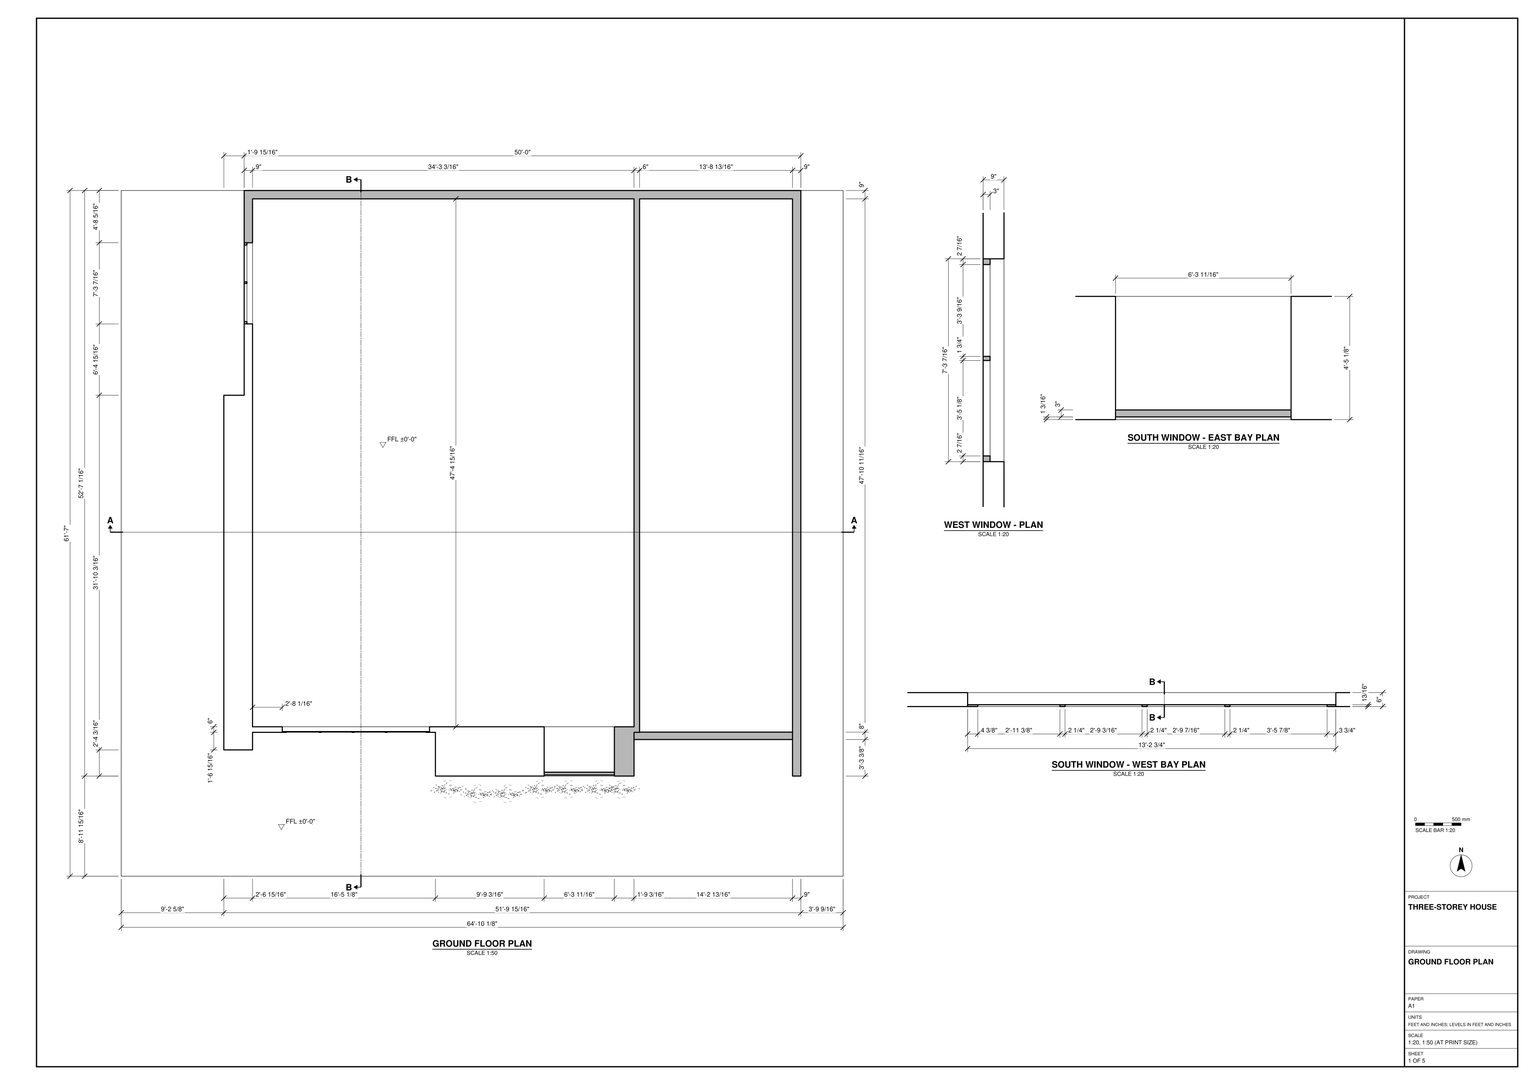
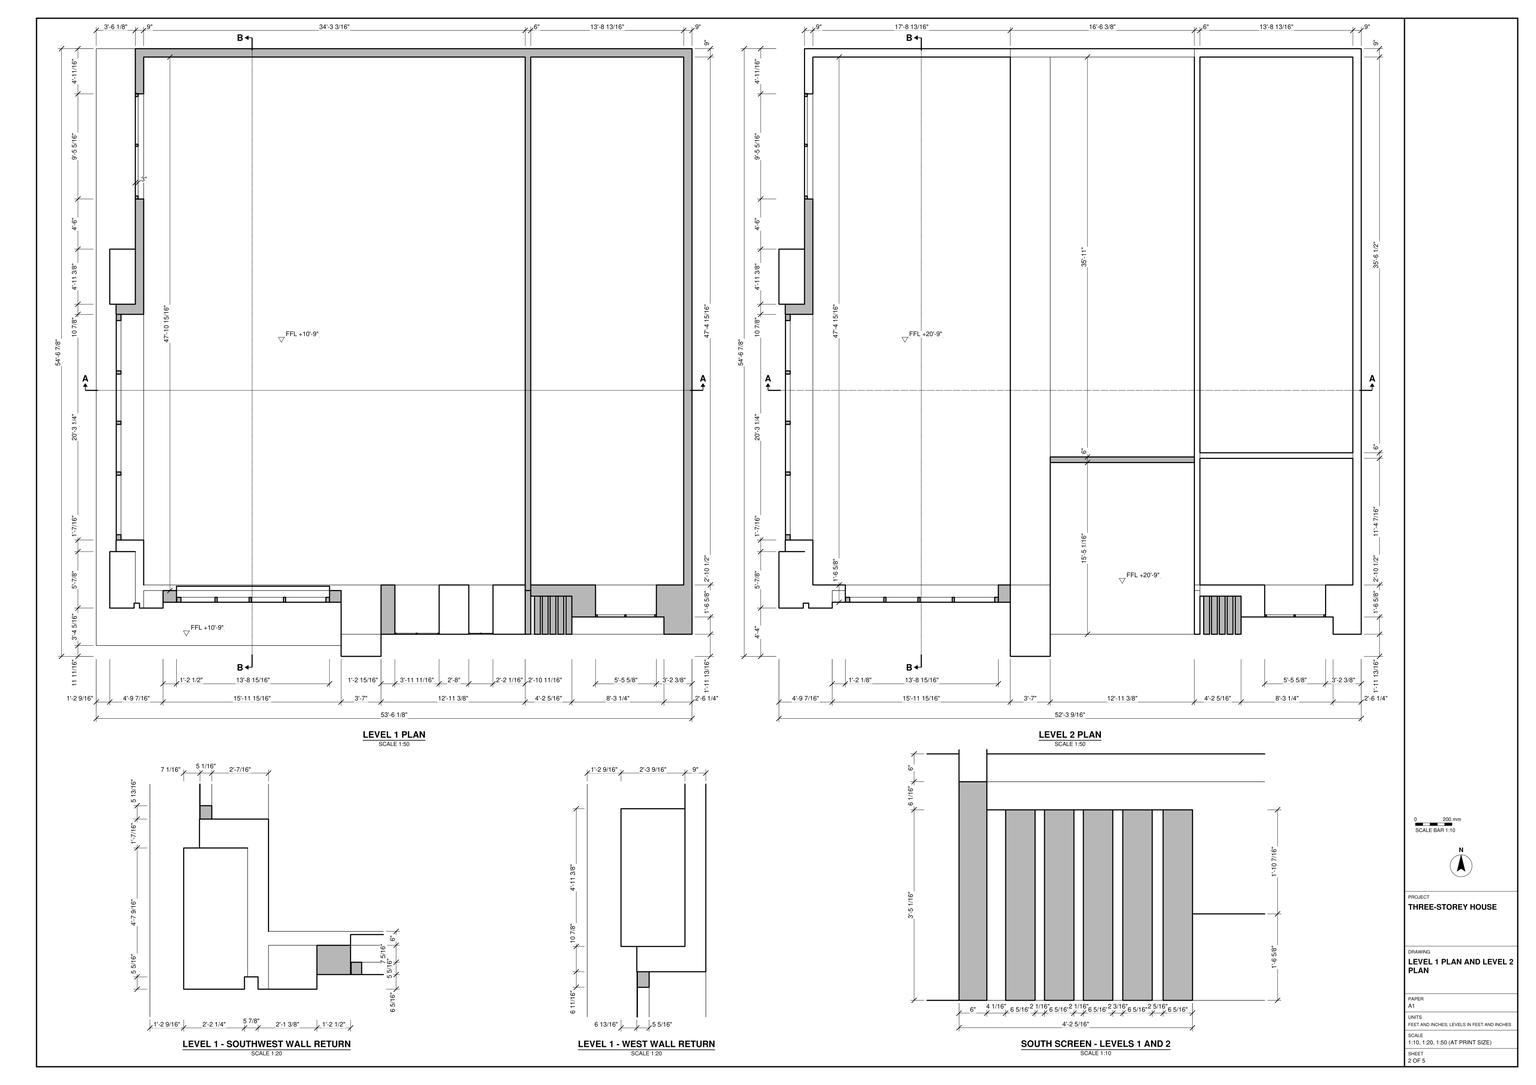
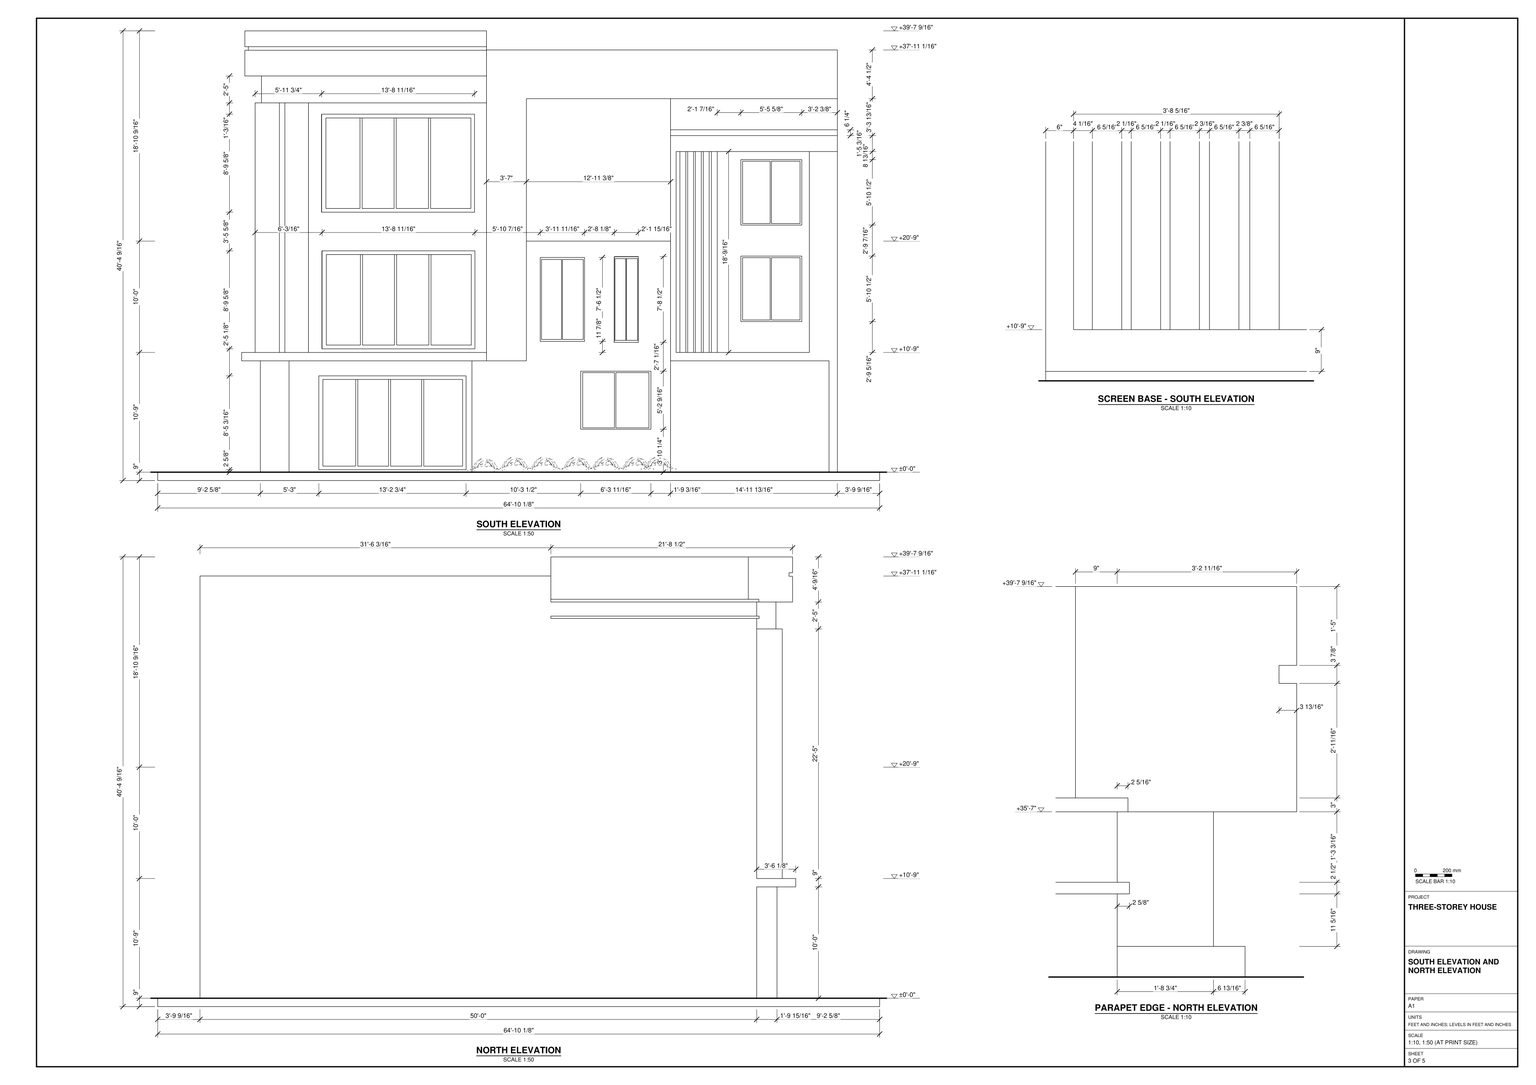
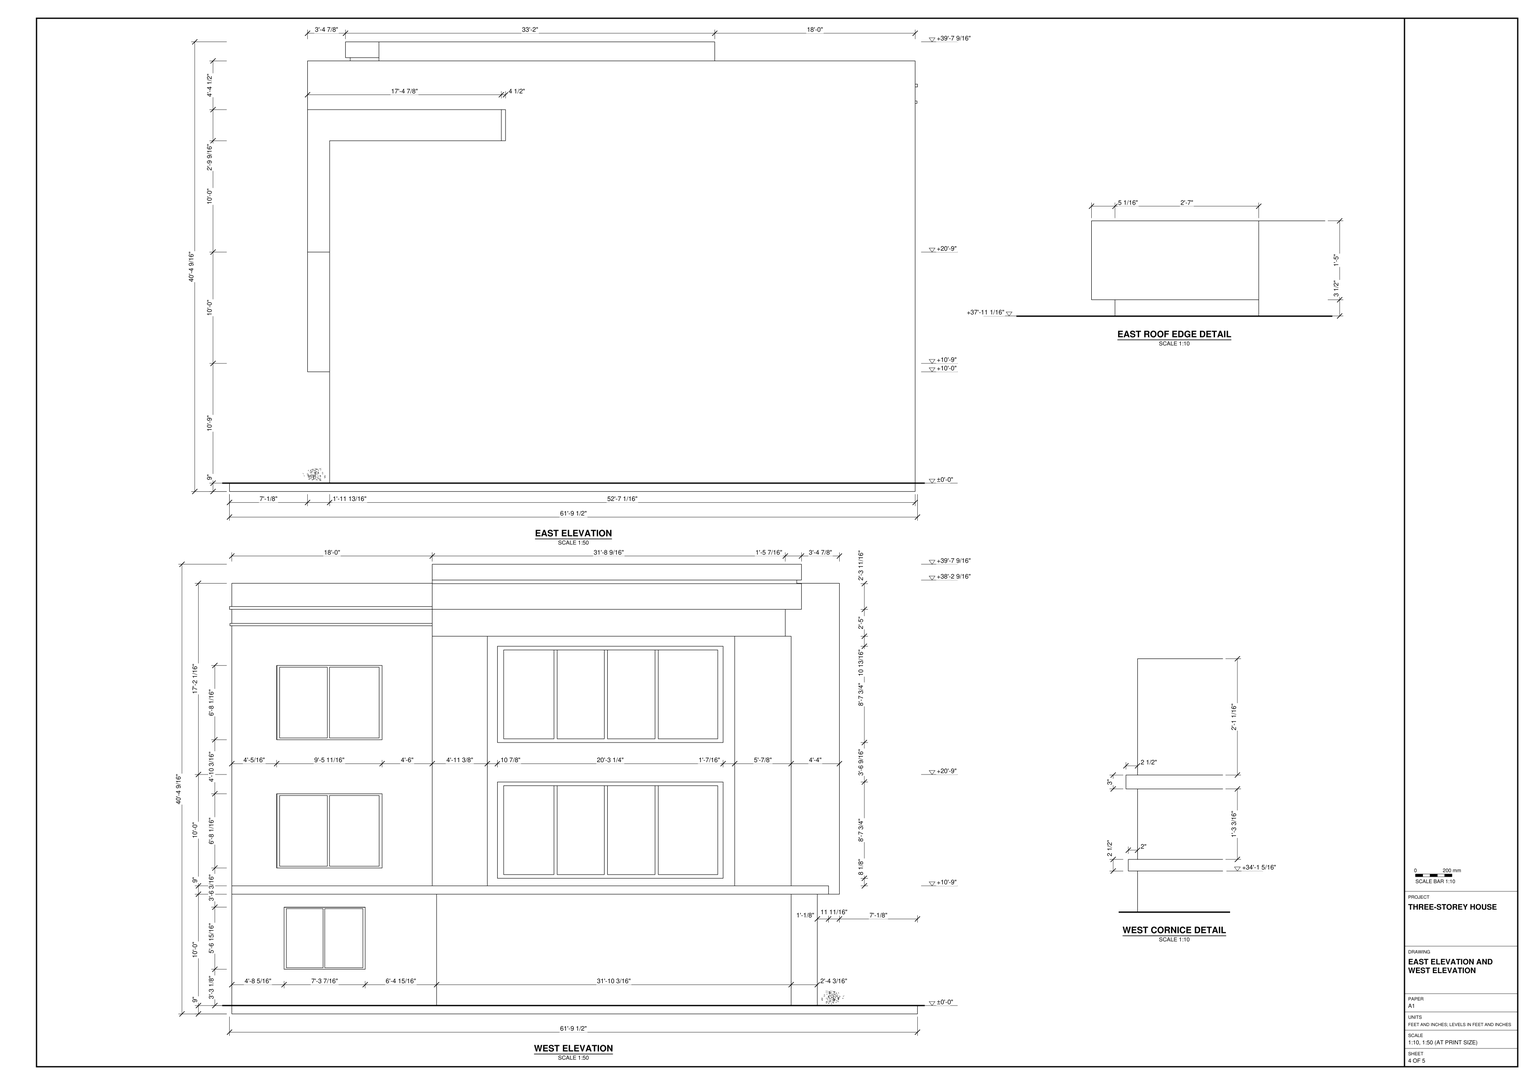
Build the three-storey house in SketchUp from task_files/diagram_01.pdf. Work in feet and inches. Including the site base, make the model 64'-10 1/8" east to west, 61'-9 1/2" north to south and 40'-4 9/16" high. Set the finished floor levels to ±0'-0", +10'-9" and +20'-9".

Use the plans to lay out the wider west bay and narrower east bay. Follow the wall thicknesses shown, including the 9" exterior walls and the 6" longitudinal dividing wall. Model the floor slabs, the stepped wall returns on the west side and the changes in depth across the south facade. Use the window details to place the frames within the openings and divide the glazing into panes. Align the wide south-facing windows in the west bay across the three storeys. In the east bay, place the vertical screen beside the upper windows, extending from its projecting base to the horizontal band above. Match the roof and parapet profiles in elevation, including the higher cap over the west bay.

Keep walls, slabs and roof elements in separate groups or components, and do the same for each furniture or joinery piece shown. Use components for repeated parts. Decor and loose items, including planting, may be any suitable library components. Save one SketchUp model as output_files/three_storey_house_with_a_screened_south_facade.skp.

# SketchUp Ruby script. Lengths in inches.
U = 1.inch
M = Sketchup.active_model
def pt(a) = Geom::Point3d.new(a.map { |v| v * U })
def face(e, loops, mat)
  f = e.add_face(loops[0].map { |a| pt(a) })
  loops[1..].each { |l| e.add_face(l.map { |a| pt(a) }).erase! }
  f.material = f.back_material = mat if mat
  f
end
# faces: each face lists its corners as indices into pts; further lists are holes
def faces(e, pts, list, mat = nil) = list.each { |f| face(e, (f[0].is_a?(Array) ? f : [f]).map { |l| l.map { |i| pts[i] } }, mat) }
# xy, xz, yz: faces in a plane at the given z, y or x. An outline is a flat list of corners, or four numbers for a rectangle; further outlines are holes
def ring(l) = l.size == 4 ? [[l[0], l[1]], [l[2], l[1]], [l[2], l[3]], [l[0], l[3]]] : l.each_slice(2).to_a
def flat(e, list, mat, &to3) = list.each { |f| face(e, (f[0].is_a?(Array) ? f : [f]).map { |l| ring(l).map { |u, v| to3.(u, v) } }, mat) }
def xy(e, z, list, mat = nil) = flat(e, list, mat) { |x, y| [x, y, z] }
def xz(e, y, list, mat = nil) = flat(e, list, mat) { |x, z| [x, y, z] }
def yz(e, x, list, mat = nil) = flat(e, list, mat) { |y, z| [x, y, z] }
def lines(e, pts, list) = list.each { |a, b| e.add_line(pt(pts[a]), pt(pts[b])) }
# prism: a flat outline (further loops are holes) pulled along v
def prism(e, loops, v, mat = nil)
  f = face(e, loops, mat); d = Geom::Vector3d.new(v.map { |x| x * U })
  f.pushpull(f.normal.samedirection?(d) ? d.length : -d.length)
end
def box(e, o, s, mat = nil) = prism(e, [[o, [o[0] + s[0], o[1], o[2]], [o[0] + s[0], o[1] + s[1], o[2]], [o[0], o[1] + s[1], o[2]]]], [0, 0, s[2]], mat)
def at(x, y, z, deg = 0) = Geom::Transformation.translation(pt([x, y, z])) * Geom::Transformation.rotation(ORIGIN, Z_AXIS, deg.degrees)
def axes(o, x, y, z) = Geom::Transformation.new([*x, 0, *y, 0, *z, 0, *pt(o).to_a, 1])
def part(name) = M.definitions.add(name)
# library, detail: a bought-in or finely detailed component or shape, given as its bounding box
def library(name, o, s) = part(name).tap { |d| box(d.entities, o, s) }
def detail(e, o, s) = box(e.add_group.entities, o, s)
def put(e, d, t, mat = nil) = e.add_instance(d, t).tap { |i| i.material = mat if mat }
def group(e, t, mat = nil) = e.add_group.tap { |g| g.transformation = t; g.material = mat if mat }.entities
root = M.entities
M.materials.add("Leaf_Half_Top_007").color = [114, 127, 96]
M.materials.add("[0009_Linen]").color = [250, 240, 230]
M.materials.add("[0028_AntiqueWhite]").color = [250, 235, 215]
M.materials.add("[Asphalt_New]").color = [58, 58, 58]
M.materials.add("[Color M00]").color = [255, 255, 255]
M.materials.add("[Color M07]").color = [58, 58, 58]
M.materials.add("[Color_F18]").color = [71, 102, 40]
M.materials.add("[Granite Light Gray]").color = [149, 148, 144]
M.materials.add("[Groundcover_Wood_Mix]").color = [22, 20, 19]
M.materials.add("[Metal Corrugated Shiny]").color = [193, 193, 97]
M.materials.add("[Pavers Flagstone Gray]").color = [162, 162, 162]
M.materials.add("[Translucent Glass Gray]").color = [128, 128, 128]
M.materials["[Translucent Glass Gray]"].alpha = 0.5
M.materials.add("[Wood Bamboo]").color = [177, 105, 43]
M.materials.add("[Wood Cherry Original]").color = [152, 86, 42]
M.materials.add("[Wood Veneer 01]").color = [120, 70, 37]
c1 = part("Pot Half 03")
p = [[1.24,1.853,0],[6.161,1.853,0],[6.586,1.426,3.732],[0.815,1.426,3.732],[1.24,1.851,0],[6.161,7.34,0],
  [6.586,7.767,3.732],[6.679,1.345,4.342],[0.722,1.345,4.342],[6.679,7.848,4.342],[6.772,1.24,4.958],[0.629,1.24,4.958],
  [6.772,7.953,4.958],[6.906,1.118,5.538],[0.495,1.118,5.538],[6.906,8.075,5.538],[7.045,0.967,6.137],[0.356,0.967,6.137],
  [7.045,8.226,6.137],[7.221,0.804,6.691],[0.18,0.804,6.691],[7.221,8.389,6.691],[7.401,0.616,7.25],[0,0.616,7.25],
  [7.401,8.577,7.25]]
faces(c1.entities,p,[[0,1,2,3],[3,0,4],[5,6,2,1],[7,8,3,2],[9,7,2,6],[10,11,8,7],[12,10,7,9],[13,14,11,10],
  [15,13,10,12],[16,17,14,13],[18,16,13,15],[19,20,17,16],[21,19,16,18],[22,23,20,19],[24,22,19,21]],"[Asphalt_New]")
c2 = part("Dirt 003")
xy(c2.entities,-0.75,[[0,-3.72,3.43,-3.72,3.43,0],[-3.43,0,0,3.72,-3.43,3.72]])
p = [[-3.43,-3.72,-0.75],[0,0,0],[-3.43,0,-0.75],[0,-3.72,-0.75],[3.43,0,-0.75],[0,3.72,-0.75],
  [3.43,3.72,-0.75]]
faces(c2.entities,p,[[0,1,2],[0,3,1],[3,4,1],[2,1,5],[1,4,6],[1,6,5]])
c3 = part("Planter Box 01")
put(c3.entities,c1,axes([-30.22,-0.62,-6.86],[4.97512,0,0],[0,1,0],[0,0,1]),"[Asphalt_New]")
put(c3.entities,c1,axes([6.66,8.58,-6.86],[-4.97512,0,0],[0,-1,0],[0,0,1]))
put(c3.entities,c2,axes([-11.66,3.97,0.41],[4.97512,0,0],[0,1,0],[0,0,1]),"[Groundcover_Wood_Mix]")
c4 = part("Group8\#1")
p = [[88.35,32.45,7.18],[88.36,32.39,7.24],[86.45,32.02,7.22],[86.4375,32.08,7.17],[88.36,32.39,7.32],[86.45,32.02,7.3],
  [88.33,32.52,7.2],[86.42,32.16,7.1875],[88.32,32.56,7.28],[86.42,32.19,7.26],[90.24,33.16,7.22],[90.27,33.09,7.2],
  [90.29,33.02,7.26],[90.29,33.02,7.34],[90.23,33.19,7.3],[88.34,32.45,7.37],[86.4375,32.08,7.35],[88.32,32.52,7.35],
  [86.42,32.16,7.34],[90.27,33.08,7.39],[90.24,33.16,7.37]]
faces(c4.entities,p,[[0,1,2,3],[1,4,5,2],[6,0,3,7],[8,6,7,9],[10,11,0,6],[11,12,1,0],[12,13,4,1],[14,10,6,8],
  [4,15,16,5],[15,17,18,16],[17,8,9,18],[13,19,15,4],[19,20,17,15],[20,14,8,17]],"[Color_F18]")
c5 = part("Stem Segment 03")
put(c5.entities,c4,at(-88.34,-32.47,-7.28))
c6 = part("Leaf Stem 003")
p = [[2.85,0.02,0.06],[2.46,0.65,0.09],[2.46,0.65,0.03],[2.85,0.02,0.02],[2.92,0.03,0.01],[2.53,0.71,0.01],
  [2.55,0.72,0.0625],[2.93,0.04,0.04],[2.49,0.68,0],[2.89,0.01,0],[2.92,0.03,0.07],[2.53,0.71,0.11],
  [1.77,1.25,0.09],[1.77,1.25,0.03],[2.46,0.65,0.09],[1.8,1.29,0],[1.83,1.33,0.01],[1.84,1.35,0.0625],
  [1.38,1.49,0.09],[1.38,1.49,0.03],[1.43,1.57,0.01],[1.44,1.59,0.0625],[1.4,1.52,0],[0.375,2.11,0.09],
  [0.375,2.11,0.03],[0.39,2.15,0],[0.42,2.19,0.01],[0.43,2.22,0.0625],[0,2.29,0.05],[0.02,2.35,0],
  [0,2.29,0.13],[0,2.29,0.09],[0.04,2.43,0.02],[0.06,2.46,0.09],[2.49,0.68,0.12],[2.89,0.01,0.08],
  [1.83,1.33,0.11],[1.8,1.29,0.12],[1.4,1.52,0.12],[1.43,1.57,0.11],[0.42,2.19,0.11],[0.39,2.15,0.12],
  [0.02,2.35,0.1875],[0.04,2.43,0.17]]
faces(c6.entities,p,[[0,1,2,3],[4,5,6,7],[8,5,4,9],[10,7,6,11],[9,3,2,8],[12,13,2,14],[2,13,8],[15,8,13],
  [8,15,5],[16,5,15],[17,6,16],[5,16,6],[13,12,18,19],[17,16,20,21],[16,15,22,20],[15,13,19,22],
  [19,18,23,24],[22,19,24,25],[20,22,25,26],[21,20,26,27],[24,28,25],[29,25,28],[25,29,26],[30,31,28,24,23],
  [32,26,29],[33,27,32],[26,32,27],[34,35,10,11],[11,6,36],[17,36,6],[34,11,37],[36,37,11],
  [37,12,34],[14,34,12],[12,37,38,18],[37,36,39,38],[36,17,21,39],[38,39,40,41],[18,38,41,23],[39,21,27,40],
  [41,40,42],[30,23,41,42],[43,42,40],[40,27,43],[33,43,27]],"[Color_F18]")
c7 = part("Leaf stalk")
put(c7.entities,c6,at(0,0,0),"[Color_F18]")
c8 = part("Leaf Half 003\#2")
xz(c8.entities,0,[[5.394,0.387,3.719,3.029,4.031,3.19,4.352,3.332,4.681,3.455,5.017,3.558,5.359,3.64,5.704,3.702,6.053,3.743,6.404,3.763,6.755,3.762,6.968,3.765,7.18,3.761,7.392,3.75,7.604,3.731,7.815,3.706,8.025,3.674,8.234,3.635,8.442,3.589,8.648,3.537,8.852,3.478,9.054,3.412,9.254,3.339,9.523,3.226,9.776,3.081,10.009,2.905,10.218,2.701,10.4,2.473,10.553,2.224,10.674,1.959,10.76,1.68,10.803,1.439,10.807,1.344,10.806,1.249,10.8,1.154,10.788,1.059,10.772,0.965,10.749,0.873,10.722,0.781,10.689,0.69,10.652,0.602,10.609,0.515,10.562,0.43,10.535,0.387]],"Leaf_Half_Top_007")
p = [[0.878,-0.545,0.444],[0.896,-0.538,0.464],[0.931,-0.525,0.507],[0.966,-0.512,0.549],[1.39,-0.366,0.995],[1.791,-0.364,0.444],
  [2.095,-0.165,1.727],[1.842,-0.358,0.429],[1.796,-0.364,0.437],[2.997,-0.164,0.429],[2.858,-0.042,2.43],[3.012,-0.163,0.428],
  [4.203,-0.043,0.406],[2.861,-0.041,2.432],[3.719,0,3.029],[5.394,0,0.387],[2.302,-0.122,1.934],[2.485,-0.09,2.102],
  [2.671,-0.064,2.268],[3.132,-0.018,2.649],[3.418,-0.005,2.848]]
faces(c8.entities,p,[[0,1,2,3,4,5],[5,4,6,7,8],[7,6,9],[9,6,10,11],[11,10,12],[10,13,14,12],[15,12,14],[16,10,6],
  [17,10,16],[18,10,17],[19,14,13],[20,14,19]],"Leaf_Half_Top_007")
c9 = part("Leaf  003")
put(c9.entities,c8,axes([0.38,-0.76,0.25],[-0.73627,0.51406,-0.06038],[0.07956,0.22794,0.97042],[-0.56957,-0.78855,0.23191]))
put(c9.entities,c8,axes([-0.33,-1.74,0.14],[-0.71206,0.54726,-0.05889],[-0.2936,-0.28379,0.91283],[0.5365,0.74143,0.40305]))
c10 = part("Stem 03")
put(c10.entities,c5,axes([-3.94,-0.51,0],[1.00831,0.3173,0.48929],[0.62823,-0.33003,-1.08062],[-0.15419,1.18746,-0.4523]))
put(c10.entities,c5,axes([3.49,-0.02,-2.22],[0.59576,-0.02646,-0.80273],[0.76313,-0.29296,0.57602],[-0.25041,-0.95576,-0.15434]))
put(c10.entities,c5,axes([9.375,1.32,-6.76],[0.76506,0.42795,-0.48118],[0.54249,-0.02572,0.83967],[0.34696,-0.90343,-0.25184]))
put(c10.entities,c5,axes([6.35,0.02,-4.79],[0.59576,-0.02646,-0.80273],[0.35669,0.9042,0.23492],[0.71961,-0.42629,0.54812]))
put(c10.entities,c5,axes([12.62,2.51,-7.16],[0.6803,0.33788,-0.02508],[0.33232,-0.6545,0.19696],[0.06597,-0.18727,-0.73361]),"[Color_F18]")
put(c10.entities,c5,axes([0.3,0.04,-0.21],[-0.84454,-0.08139,0.52927],[-0.53545,0.11632,-0.83652],[0.00652,-0.98987,-0.14182]))
put(c10.entities,c7,axes([-1.3125,-1.96,2.02],[0.30666,0.85318,0.66121],[-0.04993,0.77839,-0.74104],[-2.0519,0.10857,0.11685]))
put(c10.entities,c7,axes([-4.65,-2.32,1.92],[0.24338,0.85318,0.71076],[0.37608,0.73871,-0.80238],[-1.59205,0.25393,-0.07463]))
put(c10.entities,c7,axes([-7.2,-3.29,1.22],[0.30238,0.83595,0.58629],[0.37608,0.73871,-0.65859],[-1.58433,0.30016,-0.01484]))
put(c10.entities,c7,axes([0.53,-1.96,0.51],[0.32572,0.6177,0.78674],[-0.09946,0.84405,-0.28154],[-1.60731,-0.00658,0.27494]))
put(c10.entities,c7,axes([3.92,-1.49,-0.93],[0.30617,0.58064,0.73954],[-0.72502,0.69723,-0.01619],[-1.09889,-0.4139,0.62826]))
put(c10.entities,c7,axes([4.9375,-1.13,-0.64],[0.15705,0.93505,0.23221],[-0.515,0.47073,-0.69124],[-1.33185,0.0406,0.34107]))
put(c10.entities,c7,axes([6.62,-2.02,-3.44],[0.25326,0.61577,0.6588],[-0.59973,0.73941,-0.01442],[-0.90899,-0.43895,0.55966]))
put(c10.entities,c7,axes([7.8,1.95,-4.46],[0.47026,-0.74247,0.15265],[-0.05932,-0.60353,-0.69183],[0.55983,0.33909,-0.83034]))
put(c10.entities,c7,axes([8.1,0.54,-5.54],[0.44324,0.59809,0.36462],[0.53568,0.30234,-0.47352],[-0.95326,0.41061,-0.31748]))
put(c10.entities,c7,axes([9.91,3.23,-5.95],[0.66281,-0.36564,0.35664],[0.55741,-0.47264,-0.48381],[0.53295,0.52862,-0.61482]))
put(c10.entities,c7,axes([13.4375,2.48,-5.88],[0.62226,-0.02903,-0.01582],[0.2868,0.07076,-0.50026],[-0.12016,0.85017,-0.2373]))
put(c10.entities,c9,axes([14.48,0.92,-5.23],[0.0087,-0.21722,0.04751],[0.21837,-0.00716,-0.09125],[0.14863,0.04515,0.19139]))
put(c10.entities,c9,axes([9.9,3.39,-4.35],[-0.29123,0.01957,0.06847],[-0.02535,-0.26587,-0.00841],[0.07568,-0.01372,0.26066]))
put(c10.entities,c9,axes([7.01,1.24,-3.35],[-0.21895,-0.20956,0.10962],[0.2232,-0.10618,-0.07961],[0.2062,0.0234,0.22464]))
put(c10.entities,c9,axes([9.1,-1.16,-2.97],[0.16646,-0.16408,0.06345],[0.32123,-0.02918,-0.16141],[0.19487,0.1494,0.19131]))
put(c10.entities,c9,axes([7.62,1.91,-0.74],[-0.13636,0.15771,0.21131],[-0.30082,-0.24908,0.19555],[0.22388,-0.05253,0.25505]))
put(c10.entities,c9,axes([6.63,0.34,1.27],[0.28289,-0.14866,0.08879],[0.17621,0.08243,-0.1563],[0.15509,0.20742,0.13835]))
put(c10.entities,c9,axes([5.87,-2.37,2.55],[0.24481,-0.24553,0.03382],[0.13933,0.2091,-0.24174],[0.19372,0.29074,0.28289]))
put(c10.entities,c9,axes([2.0625,1.79,5.35],[-0.18104,0.18123,0.28972],[-0.43052,-0.16317,-0.07437],[0.10324,-0.22668,0.29612]))
put(c10.entities,c9,axes([1.29,-0.99,6.37],[0.35078,-0.04064,0.25637],[0.22081,0.3154,-0.13622],[-0.24663,0.21043,0.25293]))
put(c10.entities,c7,axes([-3.94,-4.26,-2.18],[0.2039,-0.7121,1.03293],[-0.70199,1.01563,0.56503],[-1.36054,-0.65537,-0.37049]))
c11 = part("3D Plant 003")
put(c11.entities,c3,axes([2.34,-3.97,-0.41],[0.201,0,0],[0,1,0],[0,0,1]))
put(c11.entities,c10,axes([5.43,0.67,0.04],[0.90233,-0.11399,0],[0.12659,1.00204,0],[0,0,1]))
put(c11.entities,c10,axes([4.56,-0.51,-0.05],[0.64048,0.07982,0.02703],[0.12375,-0.99231,-0.00197],[-0.04128,-0.00713,0.99912]))
put(c11.entities,c10,axes([-4.94,1.31,0.19],[-0.72845,-0.05489,0.02686],[-0.09535,1.18483,-0.16456],[0.02598,0.13957,0.98987]))
put(c11.entities,c10,axes([-5.64,-0.91,0.07],[-0.88284,0.04315,-0.01389],[-0.04884,-0.99881,0.00119],[-0.01547,0.00194,0.98988]))
put(c11.entities,c10,axes([3.75,-0.16,0.2],[0.377,-0.2222,0.04965],[0.26332,0.45308,0.02828],[-0.07969,0.00668,0.63498]))
put(c11.entities,c10,axes([-3.77,0.34,0.13],[-0.41282,0.07246,0.03267],[-0.09028,-0.51695,0.00573],[0.05019,-0.00169,0.63803]))
put(c11.entities,c10,axes([-3.89,-2.29,0.13],[-0.43617,-0.01963,0.05782],[0.02879,-0.5225,0.03978],[0.0815,0.05265,0.6326]))
put(c11.entities,c10,axes([3.46,-1.51,0.15],[0.34649,-0.00968,0.11609],[-0.02228,-0.52383,0.02283],[-0.16372,0.02836,0.49105]))
put(c11.entities,c9,axes([-3.23,-10.97,0.92],[0.14719,-0.61301,-0.08966],[0.60937,0.12663,0.13459],[-0.11174,-0.11691,0.6159]))
put(c11.entities,c9,axes([3.22,-9.64,-1.72],[0.47123,-0.37571,-0.20559],[0.42416,0.3671,0.30134],[-0.05927,-0.35994,0.52193]))
put(c11.entities,c9,axes([0.79,-6.4375,1.4375],[0.21976,-0.38322,0.22587],[0.34942,0.30462,0.17686],[-0.27528,0.08073,0.40481]))
put(c11.entities,c9,axes([1.99,4.79,6.88],[-0.22806,0.40163,0.2359],[-0.48816,-0.16923,-0.16491],[-0.06681,-0.43854,0.27612]))
put(c11.entities,c9,axes([-5.22,3.625,7.43],[-0.47836,-0.1205,0.2836],[-0.03228,-0.53536,-0.2994],[0.3042,-0.26534,0.41616]))
put(c11.entities,c9,axes([-2.24,-5.2,5.32],[0.19023,-0.33022,0.3177],[0.44902,0.20297,-0.05789],[-0.09143,0.30972,0.37668]))
put(c11.entities,c9,axes([3.33,-0.44,5.29],[0.46715,-0.167,0.15853],[-0.081,-0.39547,-0.27311],[-0.27014,-0.20951,0.34065]))
put(c11.entities,c9,axes([6.9,-4.43,-0.17],[0.51342,-0.02023,0.07039],[-0.0428,0.28715,0.45809],[-0.24354,-0.33353,0.32011]))
put(c11.entities,c9,axes([-6.28,-3.56,1.22],[-0.63664,-0.02023,0.07039],[0.05307,0.28715,0.45809],[0.30199,-0.33353,0.32011]))
put(c11.entities,c9,axes([0.92,-0.57,3.76],[-0.19279,0.26754,0.24313],[-0.36734,-0.21658,-0.04151],[0.07959,-0.3505,0.20299]))
put(c11.entities,c9,axes([-3.42,9.06,-2.66],[0.1891,0.43607,-0.42375],[0.60746,-0.11599,0.15173],[-0.02672,0.44931,0.45044]))
put(c11.entities,c9,axes([2.95,9.4,-1.4375],[0.42849,0.29992,-0.18263],[0.40356,-0.42673,0.24603],[0.00748,0.32333,0.54853]))
put(c11.entities,c9,axes([-2.67,6.99,2.51],[-0.57491,0.28187,-0.02654],[-0.2288,-0.49271,0.00048],[0.15861,-0.20895,0.48589]))
c12 = part("3D Indoor Plant 003")
put(c12.entities,c11,at(82.96,35.97,7.26),"[Asphalt_New]")
c13 = part("Group\#1")
xy(c13.entities,0,[[0,0,65.6875,2.25]],"[Color M07]")
xy(c13.entities,1.85,[[1.85,0,31.59,2.25],[32.93,0,63.84,2.25]],"[Color M07]")
xy(c13.entities,75.71,[[1.85,0,31.59,2.25],[32.93,0,63.84,2.25]],"[Color M07]")
xy(c13.entities,77.5625,[[0,0,65.6875,2.25]],"[Color M07]")
xz(c13.entities,0,[[[0,0,65.6875,77.5625],[32.93,1.85,63.84,75.71],[1.85,1.85,31.59,75.71]]],"[Color M07]")
xz(c13.entities,0,[[1.85,1.85,31.59,75.71],[32.93,1.85,63.84,75.71]],"[Translucent Glass Gray]")
xz(c13.entities,2.25,[[[0,0,65.6875,77.5625],[32.93,1.85,63.84,75.71],[1.85,1.85,31.59,75.71]]],"[Color M07]")
yz(c13.entities,0,[[0,0,2.25,77.5625]],"[Color M07]")
yz(c13.entities,1.85,[[0,1.85,2.25,75.71]],"[Color M07]")
yz(c13.entities,31.59,[[0,1.85,2.25,75.71]],"[Color M07]")
yz(c13.entities,32.93,[[0,1.85,2.25,75.71]],"[Color M07]")
yz(c13.entities,63.84,[[0,1.85,2.25,75.71]],"[Color M07]")
yz(c13.entities,65.6875,[[0,0,2.25,77.5625]],"[Color M07]")
c14 = part("Group\#2")
xy(c14.entities,0,[[0,0,99.21,5.3125]],"[Color M07]")
xy(c14.entities,2.74,[[2.74,0,24.86,5.3125],[26.26,0,46.98,5.3125],[48.38,0,69.3,5.3125],[70.7,0,96.86,5.3125]],"[Color M07]")
xy(c14.entities,68.64,[[2.74,0,24.86,5.3125],[24.86,0,26.26,0.0625],[26.26,0,46.98,5.3125],[46.98,0,48.38,0.0625],[48.38,0,69.3,5.3125],
  [69.3,0,70.7,0.0625],[70.7,0,96.86,5.3125],[24.86,0.0625,26.26,5.3125],[46.98,0.0625,48.38,5.3125],[69.3,0.0625,70.7,5.3125]],"[Color M07]")
xy(c14.entities,71.375,[[0,0,99.21,5.3125]],"[Color M07]")
xz(c14.entities,0,[[[0,0,99.21,71.375],[2.74,2.74,2.74,68.64,96.86,68.64,96.86,2.74,70.7,2.74,70.7,68.64,69.3,68.64,69.3,2.74,48.38,2.74,48.38,68.64,46.98,68.64,46.98,2.74,26.26,2.74,26.26,68.64,24.86,68.64,24.86,2.74]]],"[Color M07]")
xz(c14.entities,0,[[2.74,2.74,24.86,68.64],[26.26,2.74,46.98,68.64],[48.38,2.74,69.3,68.64],[70.7,2.74,96.86,68.64]],"[Translucent Glass Gray]")
xz(c14.entities,5.3125,[[[0,0,99.21,71.375],[2.74,2.74,2.74,68.64,96.86,68.64,96.86,2.74,70.7,2.74,70.7,68.64,69.3,68.64,69.3,2.74,48.38,2.74,48.38,68.64,46.98,68.64,46.98,2.74,26.26,2.74,26.26,68.64,24.86,68.64,24.86,2.74]]],"[Color M07]")
yz(c14.entities,0,[[0,0,5.3125,71.375]],"[Color M07]")
yz(c14.entities,2.74,[[0,2.74,5.3125,68.64]],"[Color M07]")
yz(c14.entities,24.86,[[0,2.74,5.3125,68.64]],"[Color M07]")
yz(c14.entities,26.26,[[0,2.74,5.3125,68.64]],"[Color M07]")
yz(c14.entities,46.98,[[0,2.74,5.3125,68.64]],"[Color M07]")
yz(c14.entities,48.38,[[0,2.74,5.3125,68.64]],"[Color M07]")
yz(c14.entities,69.3,[[0,2.74,5.3125,68.64]],"[Color M07]")
yz(c14.entities,70.7,[[0,2.74,5.3125,68.64]],"[Color M07]")
yz(c14.entities,96.86,[[0,2.74,5.3125,68.64]],"[Color M07]")
yz(c14.entities,99.21,[[0,0,5.3125,71.375]],"[Color M07]")
xy(root,0,[[0,0,778.125,739]])
xy(root,9,[[[338.69,107.9375,338.69,155.0625,141.5625,155.0625,141.5625,136.14,110.625,136.14,110.625,518.3125,132.5625,518.3125,132.5625,739,732.5625,739,732.5625,107.9375,723.5625,107.9375,723.5625,730,558.75,730,558.75,155.3125,552.75,155.3125,552.75,107.9375],[141.5625,161.0625,552.75,730]],[552.75,147.3125,552.75,155.0625,558.75,155.0625,558.75,155.3125,723.5625,155.3125,723.5625,147.3125],[552.75,155.0625,558.75,155.3125],[558.75,155.3125,723.5625,730],[141.5625,161.0625,552.75,730]])
xy(root,9,[[0,0,778.125,0,778.125,739,732.5625,739,732.5625,107.9375,723.5625,107.9375,723.5625,147.3125,552.75,147.3125,552.75,107.9375,338.69,107.9375,338.69,155.0625,141.5625,155.0625,141.5625,136.14,110.625,136.14,110.625,518.3125,132.5625,518.3125,132.5625,739,0,739]],"[Pavers Flagstone Gray]")
xy(root,11.625,[[173.62,155.0625,332.37,161.0625]])
xy(root,48.1,[[132.5625,595.24,141.5625,682.68]])
xy(root,55.26,[[455.89,107.9375,531.57,161.0625]])
xy(root,112.8125,[[173.62,155.0625,332.37,161.0625]])
xy(root,114.85,[[132.5625,595.24,141.5625,682.68]])
xy(root,117.83,[[455.89,107.9375,531.57,161.0625]])
xy(root,129,[[338.69,107.9375,354.375,155.0625]])
xy(root,129,[[354.375,84.125,397.375,107.9375],[90.4375,95.8125,90.4375,739,132.5625,739,132.5625,518.3125,110.625,518.3125,110.625,136.14,141.5625,136.14,141.5625,155.0625,338.69,155.0625,338.69,107.9375,354.375,107.9375,354.375,95.8125]],"[0009_Linen]")
xy(root,129,[[552.75,107.9375,552.75,155.0625,558.75,155.0625,558.75,730,723.5625,730,723.5625,107.9375]],"[0028_AntiqueWhite]")
xy(root,130.25,[[552.75,147.3125,723.5625,147.3125,723.5625,155.3125,558.75,155.3125,558.75,155.0625,552.75,155.0625]])
xy(root,132,[[141.5625,161.0625,552.75,730]])
xy(root,138,[[603.08,126.58,702.3125,126.58,702.3125,155.0625,558.75,155.0625,558.75,149,603.08,149],[105,136.14,131.2,136.14,131.2,141.45,132.5625,141.45,132.5625,197.01,105,197.01],[141.5625,136.14,162.4375,155.0625],[162.4375,142.45,354.375,155.0625],[558.75,155.0625,723.5625,161.0625],
  [141.5625,161.0625,552.75,730],[558.75,161.0625,723.5625,730],[105,463.62,132.5625,522.99]])
xy(root,138,[[90.4375,95.8125,354.375,95.8125,354.375,142.45,162.4375,142.45,162.4375,136.14,137.0625,136.14,137.0625,141.45,131.2,141.45,131.2,136.14,105,136.14,105,197.01,111.8125,197.01,111.8125,463.62,105,463.62,105,522.99,132.5625,522.99,132.5625,739,90.4375,739],[558.75,107.9375,562.8,149],[569.14,107.9375,571.18,149],[577.52,107.9375,579.55,149],[585.89,107.9375,588.05,149],
  [594.39,107.9375,596.74,149],[603.08,107.9375,702.3125,126.58]],"[0028_AntiqueWhite]")
xy(root,138,[[562.8,107.9375,569.14,149],[571.18,107.9375,577.52,149],[579.55,107.9375,585.89,149],[588.05,107.9375,594.39,149],[596.74,107.9375,603.08,149]],"[Wood Bamboo]")
xy(root,141.93,[[176.95,142.45,341.89,155.0625],[176.95,155.0625,341.89,159.6875]])
xy(root,146.15,[[111.8125,209.47,141.5625,452.72]])
xy(root,148.86,[[491.99,107.9375,518.05,161.0625]])
xy(root,149.89,[[412.32,107.9375,460,161.0625]])
xy(root,157.21,[[132.5625,577.01,141.5625,690.32]])
xy(root,171.34,[[628.55,126.58,694.17,161.0625]])
xy(root,237.27,[[132.5625,577.01,141.5625,690.32]])
xy(root,240.39,[[412.32,107.9375,460,161.0625]])
xy(root,241.11,[[491.99,107.9375,518.05,161.0625]])
xy(root,241.84,[[628.55,126.58,694.17,161.0625]])
xy(root,247.55,[[176.95,142.45,341.89,155.0625],[176.95,155.0625,341.89,159.6875]])
xy(root,249.9,[[552.75,155.0625,558.75,155.0625,558.75,161.0625,397.375,161.0625,397.375,730,552.75,730],[141.5625,161.0625,354.375,730],[354.375,161.0625,397.375,730],[111.8125,209.47,141.5625,452.72]])
xy(root,251.8125,[[558.75,161.0625,723.5625,730]])
xy(root,258,[[552.75,155.0625,558.75,161.0625],[141.5625,161.0625,354.375,730],[354.375,161.0625,397.375,730],[558.75,161.0625,723.5625,297.51],[397.375,293,552.75,299.02],
  [558.75,297.51,723.5625,303.51],[397.375,299.02,552.75,730],[558.75,303.51,723.5625,730]])
xy(root,258,[[397.375,107.9375,552.75,107.9375,552.75,161.0625,558.75,161.0625,558.75,155.0625,552.75,155.0625,552.75,293,397.375,293]],"[0028_AntiqueWhite]")
xy(root,275.28,[[628.55,126.58,694.17,161.0625]])
xy(root,289.18,[[176.51,142.45,341.45,161.0625]])
xy(root,292.46,[[111.8125,209.47,141.5625,452.72]])
xy(root,295.46,[[132.5625,577.01,141.5625,690.32]])
xy(root,345.78,[[628.55,126.58,694.17,161.0625]])
xy(root,354.5625,[[558.75,107.9375,562.8,149],[569.14,107.9375,571.18,149],[577.52,107.9375,579.55,149],[585.89,107.9375,588.05,149],[594.39,107.9375,596.74,149],
  [603.08,107.9375,702.3125,126.58]],"[0028_AntiqueWhite]")
xy(root,372,[[558.75,161.0625,723.5625,297.51]])
xy(root,375.52,[[132.5625,577.01,141.5625,690.32]])
xy(root,378,[[552.75,107.9375,732.5625,297.51]],"[0028_AntiqueWhite]")
xy(root,394.8,[[176.51,142.45,341.45,161.0625]])
xy(root,396.21,[[111.8125,209.47,141.5625,452.72]])
xy(root,401.5625,[[141.5625,161.0625,354.375,730]])
xy(root,407,[[105,136.14,105,197.01,111.8125,197.01,111.8125,142.45,162.4375,142.45,162.4375,136.14,137.0625,136.14,137.0625,141.45,131.2,141.45,131.2,136.14],[111.8125,142.45,132.5625,197.01],[111.8125,463.62,132.5625,522.99]])
xy(root,407,[[105,463.62,111.8125,522.99]],"[Wood Cherry Original]")
xy(root,411.53,[[397.375,293,552.75,299.02],[397.375,299.02,552.75,730]])
xy(root,411.53,[[397.375,84.125,397.375,293,552.75,293,552.75,297.51,732.5625,297.51,732.5625,84.125]],"[0009_Linen]")
xy(root,418.3125,[[129.9375,522.99,129.9375,741,354.375,741,354.375,739,132.5625,739,132.5625,522.99]],"[Color M07]")
xy(root,420.8125,[[129.9375,522.99,132.5625,522.99,132.5625,739,354.375,739,354.375,741,129.9375,741]],"[Color M07]")
xy(root,436,[[111.8125,142.45,111.8125,522.99,132.5625,522.99,132.5625,739,354.375,739,354.375,730,141.5625,730,141.5625,161.0625,354.375,161.0625,354.375,142.45]])
xy(root,436,[[130.25,522.99,130.25,741.5,354.375,741.5,354.375,739,132.5625,739,132.5625,522.99]],"[Color M07]")
xy(root,436,[[93.875,125.01,93.875,522.99,111.8125,522.99,111.8125,142.45,354.375,142.45,354.375,125.01]],"[Wood Veneer 01]")
xy(root,439,[[141.5625,161.0625,354.375,161.0625,354.375,741.5,130.25,741.5,130.25,522.99,141.5625,522.99]],"[0028_AntiqueWhite]")
xy(root,463.6875,[[93.875,125.01,354.375,130.08],[93.875,130.08,97.6875,522.99]],"[Wood Veneer 01]")
xy(root,464.0625,[[354.375,84.125,732.5625,739]],"[0028_AntiqueWhite]")
xy(root,467.5625,[[93.875,125.01,93.875,522.99,97.6875,522.99,97.6875,130.08,354.375,130.08,354.375,125.01]],"[Wood Veneer 01]")
xy(root,484.5625,[[93.875,125.01,354.375,125.01,354.375,161.0625,141.5625,161.0625,141.5625,522.99,93.875,522.99]],"[Wood Veneer 01]")
xz(root,0,[[0,0,778.125,9]],"[Pavers Flagstone Gray]")
xz(root,84.125,[[354.375,129,397.375,129,397.375,411.53,732.5625,411.53,732.5625,464.0625,354.375,464.0625]],"[0028_AntiqueWhite]")
xz(root,95.8125,[[90.4375,129,354.375,138]],"[0028_AntiqueWhite]")
xz(root,107.9375,[[[338.69,9,552.75,9,552.75,258,397.375,258,397.375,129,338.69,129],[455.89,55.26,531.57,117.83],[412.32,149.89,460,240.39],[491.99,148.86,518.05,241.11]],[723.5625,9,732.5625,9,732.5625,354.5625,702.3125,354.5625,702.3125,138,558.75,138,558.75,354.5625,732.5625,354.5625,732.5625,371.75,552.75,371.75,552.75,129,723.5625,129],[552.75,371.75,732.5625,378]],"[0028_AntiqueWhite]")
xz(root,107.9375,[[562.8,138,569.14,354.5625],[571.18,138,577.52,354.5625],[579.55,138,585.89,354.5625],[588.05,138,594.39,354.5625],[596.74,138,603.08,354.5625]],"[Wood Bamboo]")
xz(root,125.01,[[93.875,436,354.375,463.6875],[93.875,467.5625,354.375,484.5625]],"[Wood Veneer 01]")
xz(root,126.58,[[[603.08,138,702.3125,354.5625],[628.55,171.34,694.17,241.84],[628.55,275.28,694.17,345.78]]],"[Color M07]")
xz(root,130.08,[[97.6875,463.6875,354.375,467.5625]],"[Wood Veneer 01]")
xz(root,136.14,[[110.625,9,141.5625,129],[105,138,131.2,407],[137.0625,138,162.4375,407]],"[0028_AntiqueWhite]")
xz(root,141.45,[[131.2,138,137.0625,407]],"[Metal Corrugated Shiny]")
xz(root,142.45,[[[162.4375,138,354.375,407],[176.51,289.18,341.45,394.8],[176.95,141.93,341.89,247.55]]],"[Color M07]")
xz(root,142.45,[[111.8125,407,354.375,436]],"[Wood Veneer 01]")
xz(root,147.3125,[[552.75,9,723.5625,130.25]],"[Color M07]")
xz(root,149,[[577.52,138,579.55,354.5625],[585.89,138,588.05,354.5625],[594.39,138,596.74,354.5625]])
xz(root,149,[[558.75,138,562.8,354.5625],[569.14,138,571.18,354.5625]],"[0028_AntiqueWhite]")
xz(root,149,[[562.8,138,569.14,354.5625],[571.18,138,577.52,354.5625],[579.55,138,585.89,354.5625],[588.05,138,594.39,354.5625],[596.74,138,603.08,354.5625]],"[Wood Bamboo]")
xz(root,155.0625,[[552.75,9,558.75,129],[141.5625,129,354.375,138],[552.75,129,558.75,130.25],[[162.4375,138,354.375,258],[176.95,141.93,341.89,247.55]],[552.75,138,558.75,249.9],
  [552.75,249.9,558.75,258]])
xz(root,155.0625,[[[141.5625,9,338.69,129],[173.62,11.625,332.37,112.8125]]],"[Granite Light Gray]")
xz(root,155.3125,[[558.75,9,723.5625,130.25]])
xz(root,159.6875,[[176.95,141.93,341.89,247.55]],"[Color M00]")
xz(root,161.0625,[[[141.5625,9,552.75,129],[173.62,11.625,332.37,112.8125],[455.89,55.26,531.57,117.83]],[141.5625,129,552.75,132],[141.5625,132,552.75,138],[[397.375,138,552.75,249.9],[412.32,149.89,460,240.39],[491.99,148.86,518.05,241.11]],[[558.75,138,723.5625,251.8125],[628.55,171.34,694.17,241.84]],
  [141.5625,249.9,354.375,258],[354.375,249.9,397.375,258],[552.75,249.9,558.75,258],[558.75,251.8125,723.5625,258],[141.5625,258,354.375,287],
  [[558.75,258,723.5625,372],[628.55,275.28,694.17,345.78]],[[141.5625,287,354.375,401.5625],[176.51,289.18,341.45,394.8]],[141.5625,401.5625,354.375,407],[141.5625,407,354.375,436],[141.5625,436,354.375,439]])
xz(root,161.0625,[[141.5625,439,354.375,484.5625]],"[Wood Veneer 01]")
xz(root,197.01,[[105,138,111.8125,407],[111.8125,138,132.5625,258],[111.8125,258,132.5625,287],[111.8125,287,132.5625,407]])
xz(root,209.47,[[111.8125,146.15,141.5625,249.9],[111.8125,292.46,141.5625,396.21]])
xz(root,293,[[397.375,258,552.75,411.53]],"[0028_AntiqueWhite]")
xz(root,297.51,[[558.75,258,723.5625,354.5625],[552.75,354.5625,558.75,371.75],[558.75,354.5625,723.5625,371.75],[552.75,371.75,558.75,378],[558.75,371.75,723.5625,372],
  [558.75,372,723.5625,378]])
xz(root,297.51,[[552.75,378,732.5625,411.53]],"[0028_AntiqueWhite]")
xz(root,299.02,[[397.375,258,552.75,411.53]])
xz(root,303.51,[[558.75,258,723.5625,378]])
xz(root,452.72,[[111.8125,146.15,141.5625,249.9],[111.8125,292.46,141.5625,396.21]])
xz(root,463.62,[[111.8125,138,132.5625,258],[111.8125,258,132.5625,287],[111.8125,287,132.5625,407]])
xz(root,463.62,[[105,138,111.8125,407]],"[Wood Cherry Original]")
xz(root,518.3125,[[110.625,9,132.5625,129]],"[0028_AntiqueWhite]")
xz(root,522.99,[[129.9375,418.3125,132.5625,420.8125],[132.5625,418.3125,141.5625,420.8125],[132.5625,420.8125,141.5625,420.8125,141.5625,439,130.25,439,130.25,436,132.5625,436]])
xz(root,522.99,[[105,138,132.5625,407]],"[Wood Cherry Original]")
xz(root,522.99,[[111.8125,407,111.8125,436,132.5625,436,132.5625,420.8125,129.9375,420.8125,129.9375,418.3125,132.5625,418.3125,132.5625,407],[93.875,436,93.875,463.6875,97.6875,463.6875,97.6875,467.5625,93.875,467.5625,93.875,484.5625,141.5625,484.5625,141.5625,439,130.25,439,130.25,436]],"[Wood Veneer 01]")
xz(root,577.01,[[132.5625,157.21,141.5625,237.27],[132.5625,295.46,141.5625,375.52]])
xz(root,595.24,[[132.5625,48.1,141.5625,114.85]])
xz(root,682.68,[[132.5625,48.1,141.5625,114.85]])
xz(root,690.32,[[132.5625,157.21,141.5625,237.27],[132.5625,295.46,141.5625,375.52]])
xz(root,730,[[141.5625,9,552.75,129],[558.75,9,723.5625,129],[141.5625,129,552.75,132],[558.75,129,723.5625,138],[141.5625,132,166.25,138],
  [166.25,132,172,138],[172,132,552.75,138],[141.5625,138,166.25,249.9],[166.25,138,172,249.9],[172,138,552.75,249.9],
  [558.75,138,723.5625,251.8125],[141.5625,249.9,166.25,258],[166.25,249.9,172,258],[172,249.9,354.375,258],[354.375,249.9,397.375,258],
  [397.375,249.9,552.75,258],[558.75,251.8125,575.9375,258],[575.9375,251.8125,723.5625,258],[141.5625,258,354.375,401.5625],[558.75,258,723.5625,378],
  [141.5625,401.5625,354.375,407],[141.5625,407,354.375,436]])
xz(root,739,[[0,0,778.125,9],[132.5625,418.3125,354.375,420.8125]])
xz(root,739,[[132.5625,9,132.5625,129,90.4375,129,90.4375,138,132.5625,138,132.5625,418.3125,354.375,418.3125,354.375,420.8125,132.5625,420.8125,132.5625,436,354.375,436,354.375,464.0625,732.5625,464.0625,732.5625,9]],"[0028_AntiqueWhite]")
xz(root,741,[[129.9375,418.3125,354.375,420.8125]],"[Color M07]")
xz(root,741.5,[[130.25,436,354.375,439]],"[Color M07]")
yz(root,0,[[0,0,739,9]],"[Pavers Flagstone Gray]")
yz(root,90.4375,[[95.8125,129,739,138]],"[0028_AntiqueWhite]")
yz(root,93.875,[[125.01,436,522.99,463.6875],[125.01,467.5625,522.99,484.5625]],"[Wood Veneer 01]")
yz(root,97.6875,[[130.08,463.6875,522.99,467.5625]],"[Wood Veneer 01]")
yz(root,105,[[136.14,138,197.01,407]],"[0028_AntiqueWhite]")
yz(root,105,[[463.62,138,522.99,407]],"[Wood Cherry Original]")
yz(root,110.625,[[136.14,9,518.3125,129]],"[0028_AntiqueWhite]")
yz(root,111.8125,[[[197.01,138,463.62,407],[209.47,146.15,452.72,249.9],[209.47,292.46,452.72,396.21]]],"[Color M07]")
yz(root,111.8125,[[142.45,407,522.99,436]],"[Wood Veneer 01]")
yz(root,129.9375,[[522.99,418.3125,741,420.8125]],"[Color M07]")
yz(root,130.25,[[522.99,436,741.5,439]],"[Color M07]")
yz(root,131.2,[[136.14,138,141.45,407]],"[Metal Corrugated Shiny]")
yz(root,132.5625,[[463.62,138,522.99,407],[522.99,418.3125,739,420.8125]])
yz(root,132.5625,[[[518.3125,9,739,129],[595.24,48.1,682.68,114.85]],[[522.99,138,739,418.3125],[577.01,157.21,690.32,237.27],[577.01,295.46,690.32,375.52]],[522.99,420.8125,739,436]],"[0028_AntiqueWhite]")
yz(root,137.0625,[[136.14,138,141.45,407]],"[Metal Corrugated Shiny]")
yz(root,141.5625,[[[161.0625,9,730,129],[595.24,48.1,682.68,114.85]],[136.14,129,155.0625,138],[161.0625,129,730,132],[161.0625,132,730,138],[[161.0625,138,730,138,730,249.9,452.72,249.9,452.72,146.15,209.47,146.15,209.47,249.9,161.0625,249.9],[577.01,157.21,690.32,237.27]],
  [161.0625,249.9,522.99,258],[522.99,249.9,730,258],[161.0625,258,522.99,287],[522.99,258,730,287],[[161.0625,287,522.99,401.5625],[209.47,292.46,452.72,396.21]],
  [[522.99,287,730,401.5625],[577.01,295.46,690.32,375.52]],[161.0625,401.5625,522.99,407],[522.99,401.5625,730,407],[161.0625,407,522.99,436],[522.99,407,730,436],
  [161.0625,436,522.99,439]])
yz(root,141.5625,[[136.14,9,155.0625,129]],"[0028_AntiqueWhite]")
yz(root,141.5625,[[161.0625,439,522.99,484.5625]],"[Wood Veneer 01]")
yz(root,162.4375,[[142.45,138,155.0625,258]])
yz(root,162.4375,[[136.14,138,142.45,407]],"[0028_AntiqueWhite]")
yz(root,173.62,[[155.0625,11.625,161.0625,112.8125]])
yz(root,176.51,[[142.45,289.18,161.0625,394.8]])
yz(root,176.95,[[142.45,141.93,155.0625,247.55],[155.0625,141.93,159.6875,247.55]])
yz(root,332.37,[[155.0625,11.625,161.0625,112.8125]])
yz(root,338.69,[[107.9375,9,155.0625,129]],"[0028_AntiqueWhite]")
yz(root,341.45,[[142.45,289.18,161.0625,394.8]])
yz(root,341.89,[[142.45,141.93,155.0625,247.55],[155.0625,141.93,159.6875,247.55]])
yz(root,354.375,[[154.9375,129,155.0625,138],[142.45,138,154.9375,258],[154.9375,138,155.0625,258],[142.45,258,154.9375,287],[154.9375,258,155.0625,287],
  [155.0625,258,161.0625,287],[161.0625,258,730,401.5625],[142.45,287,154.9375,378],[154.9375,287,155.0625,378],[155.0625,287,161.0625,407],
  [142.45,378,154.9375,407],[154.9375,378,155.0625,407],[161.0625,401.5625,730,439],[142.45,407,154.9375,436],[154.9375,407,155.0625,436],
  [155.0625,407,161.0625,436],[730,418.3125,739,420.8125],[125.01,436,154.9375,463.6875],[154.9375,436,155.0625,463.6875],[155.0625,436,161.0625,463.6875],
  [730,436,739,439],[130.08,463.6875,154.9375,464.0625],[154.9375,463.6875,155.0625,464.0625],[155.0625,463.6875,161.0625,464.0625]])
yz(root,354.375,[[84.125,129,84.125,464.0625,130.08,464.0625,130.08,463.6875,125.01,463.6875,125.01,436,142.45,436,142.45,138,95.8125,138,95.8125,129],[161.0625,439,739,464.0625]],"[0028_AntiqueWhite]")
yz(root,354.375,[[739,418.3125,741,420.8125],[739,436,741.5,439]],"[Color M07]")
yz(root,354.375,[[130.08,464.0625,161.0625,467.5625],[125.01,467.5625,161.0625,484.5625]],"[Wood Veneer 01]")
yz(root,397.375,[[107.9375,138,161.0625,258],[161.0625,249.9,730,258],[293,258,299.02,411.53]])
yz(root,397.375,[[84.125,129,107.9375,258],[84.125,258,293,411.53]],"[0028_AntiqueWhite]")
yz(root,412.32,[[107.9375,149.89,161.0625,240.39]])
yz(root,455.89,[[107.9375,55.26,161.0625,117.83]])
yz(root,460,[[107.9375,149.89,161.0625,240.39]])
yz(root,491.99,[[107.9375,148.86,161.0625,241.11]])
yz(root,518.05,[[107.9375,148.86,161.0625,241.11]])
yz(root,531.57,[[107.9375,55.26,161.0625,117.83]])
yz(root,552.75,[[147.3125,9,155.0625,129],[161.0625,9,730,129],[107.9375,129,107.9375,138,155.0625,138,155.0625,130.25,147.3125,130.25,147.3125,129],[147.3125,129,155.0625,130.25],[155.0625,129,161.0625,138],
  [161.0625,129,730,132],[161.0625,132,730,138],[107.9375,138,155.0625,249.9],[155.0625,138,161.0625,249.9],[161.0625,138,730,249.9],
  [107.9375,249.9,155.0625,258],[155.0625,249.9,161.0625,258],[161.0625,249.9,297.51,258],[297.51,249.9,730,258],[293,258,297.51,354.5625],
  [297.51,258,299.02,378],[299.02,258,730,378],[293,354.5625,297.51,371.75],[293,371.75,297.51,378],[293,378,297.51,411.53],
  [297.51,378,299.02,411.53],[299.02,378,730,411.53]])
yz(root,552.75,[[107.9375,9,147.3125,129],[107.9375,258,293,371.75],[107.9375,371.75,293,378]],"[0028_AntiqueWhite]")
yz(root,558.75,[[155.0625,9,155.3125,129],[155.3125,9,730,129],[155.0625,129,155.3125,130.25],[149,138,155.0625,249.9],[155.0625,138,161.0625,249.9],
  [161.0625,138,730,251.8125],[149,249.9,155.0625,258],[155.0625,249.9,161.0625,258],[161.0625,251.8125,730,258],[161.0625,258,297.51,372],
  [303.51,258,730,378]])
yz(root,558.75,[[107.9375,138,149,354.5625]],"[0028_AntiqueWhite]")
yz(root,562.8,[[107.9375,138,149,354.5625]],"[Wood Bamboo]")
yz(root,569.14,[[107.9375,138,149,354.5625]],"[Wood Bamboo]")
yz(root,571.18,[[107.9375,138,149,354.5625]],"[Wood Bamboo]")
yz(root,577.52,[[107.9375,138,149,354.5625]],"[Wood Bamboo]")
yz(root,579.55,[[107.9375,138,149,354.5625]],"[Wood Bamboo]")
yz(root,585.89,[[107.9375,138,149,354.5625]],"[Wood Bamboo]")
yz(root,588.05,[[107.9375,138,149,354.5625]],"[Wood Bamboo]")
yz(root,594.39,[[107.9375,138,149,354.5625]],"[Wood Bamboo]")
yz(root,596.74,[[107.9375,138,149,354.5625]],"[Wood Bamboo]")
yz(root,603.08,[[126.58,138,149,354.5625]])
yz(root,603.08,[[107.9375,138,126.58,354.5625]],"[Wood Bamboo]")
yz(root,628.55,[[126.58,171.34,161.0625,241.84],[126.58,275.28,161.0625,345.78]])
yz(root,694.17,[[126.58,171.34,161.0625,241.84],[126.58,275.28,161.0625,345.78]])
yz(root,702.3125,[[107.9375,138,126.58,354.5625]],"[0028_AntiqueWhite]")
yz(root,723.5625,[[147.3125,9,155.3125,129],[155.3125,9,730,129],[147.3125,129,155.3125,130.25],[161.0625,138,730,251.8125],[161.0625,251.8125,730,258],
  [161.0625,258,297.51,372],[303.51,258,730,378]])
yz(root,723.5625,[[107.9375,9,147.3125,129]],"[0028_AntiqueWhite]")
yz(root,732.5625,[[107.9375,9,739,9,739,464.0625,84.125,464.0625,84.125,411.53,297.51,411.53,297.51,378,107.9375,378]],"[0028_AntiqueWhite]")
yz(root,778.125,[[0,0,739,9]],"[Pavers Flagstone Gray]")
p = [[552.75,730,258],[552.75,739,258],[552.75,730,378],[552.75,739,378],[723.5625,303.51,378],[723.5625,303.51,464.0625],
  [723.5625,730,378],[723.5625,730,464.0625],[558.75,303.51,378],[558.75,303.51,464.0625],[558.75,730,378],[558.75,730,464.0625],
  [552.75,297.51,411.53],[552.75,297.51,464.0625],[723.5625,297.51,411.53],[723.5625,297.51,464.0625],[552.75,730,464.0625],[552.75,730,411.53],
  [397.375,730,464.0625],[397.375,730,411.53],[564.625,161.0625,378],[564.625,161.0625,372],[723.5625,161.0625,372],[723.5625,161.0625,378],
  [558.75,161.0625,372],[558.75,161.0625,378],[723.5625,297.51,371.75],[732.5625,297.51,371.75],[723.5625,297.51,354.5625],[732.5625,297.51,354.5625],
  [354.375,730,287],[354.375,739,287],[354.375,730,407],[354.375,739,407],[141.5625,522.99,249.9],[141.5625,522.99,248.25],
  [702.3125,155.0625,129],[702.3125,155.0625,138],[141.5625,730,436],[141.5625,730,439]]
lines(root,p,[[0,1],[2,3],[4,5],[6,7],[8,9],[10,11],[12,13],[14,15],[16,17],[18,19],[20,21],[22,23],
  [24,25],[26,27],[28,29],[30,31],[32,33],[34,35],[36,37],[38,39]])
put(root,c12,at(269.73,58.25,9))
put(root,c12,at(301.76,53.35,10.48))
put(root,c12,at(334.13,53.35,10.48))
put(root,c12,at(369,58.11,10.48))
put(root,c12,at(399.9375,58.11,10.48))
put(root,c12,at(432.5625,58.11,10.48))
put(root,c12,at(456.6875,58.11,10.48))
put(root,c13,axes([455.89,109.1,55.26],[1.15224,0,0],[0,1.332,0],[0,0,0.8064]))
put(root,c14,axes([177.19,142.45,141.93],[1.66,0,0],[0,1,0],[0,0,1.47986]))
put(root,c13,axes([628.55,126.58,171.34],[0.99905,0,0],[0,1.02564,0],[0,0,0.90894]))
put(root,c13,axes([628.55,126.58,275.28],[0.99905,0,0],[0,1.02564,0],[0,0,0.90894]))
put(root,c13,axes([412.32,107.9375,149.89],[0.72598,0,0],[0,0.51282,0],[0,0,1.1668]))
put(root,c13,axes([492.13,108.18,148.86],[0.39462,0,0],[0,0.40513,0],[0,0,1.1922]))
put(root,c14,axes([176.75,142.45,289.18],[1.66,0,0],[0,1,0],[0,0,1.47986]))
put(root,c14,axes([112.02,452.72,146.15],[0,-2.45178,0],[0.96,0,0],[0,0,1.45359]))
put(root,c14,axes([112.02,452.72,292.46],[0,-2.45178,0],[0.96,0,0],[0,0,1.45359]))
put(root,c14,axes([173.62,155.86,11.625],[1.60008,0,0],[0,-0.15,0],[0,0,1.41769]))
put(root,c13,axes([132.5625,682.68,48.1],[0,-1.33111,0],[1.332,0,0],[0,0,0.86285]))
put(root,c13,axes([132.5625,690.68,157.21],[0,-1.73045,0],[1.332,0,0],[0,0,1.03223]))
put(root,c13,axes([132.5625,690.68,295.46],[0,-1.73045,0],[1.332,0,0],[0,0,1.03223]))
